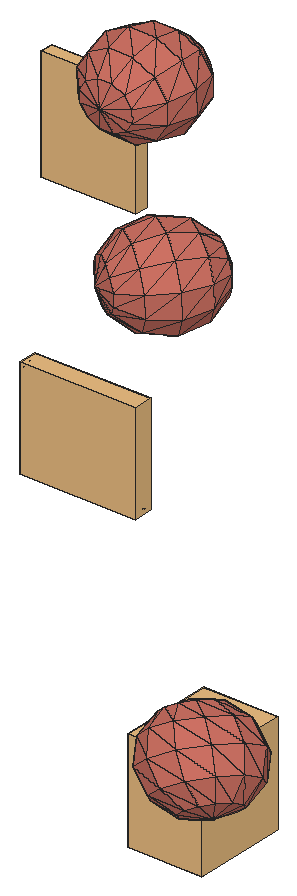
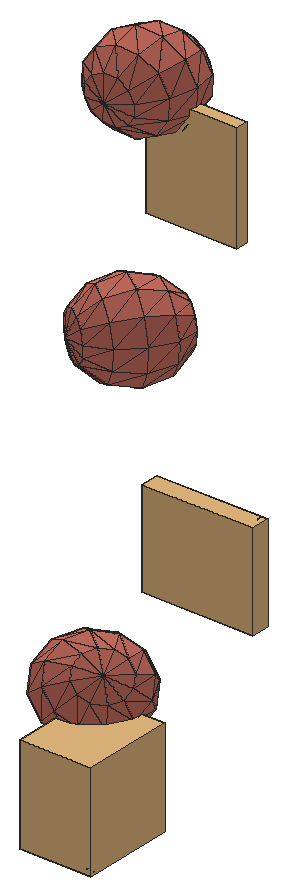
# SketchUp Ruby script. Lengths in inches.
U = 1.inch
M = Sketchup.active_model
def pt(a) = Geom::Point3d.new(a.map { |v| v * U })
def face(e, loops, mat)
  f = e.add_face(loops[0].map { |a| pt(a) })
  loops[1..].each { |l| e.add_face(l.map { |a| pt(a) }).erase! }
  f.material = f.back_material = mat if mat
  f
end
# faces: each face lists its corners as indices into pts; further lists are holes
def faces(e, pts, list, mat = nil) = list.each { |f| face(e, (f[0].is_a?(Array) ? f : [f]).map { |l| l.map { |i| pts[i] } }, mat) }
# xy, xz, yz: faces in a plane at the given z, y or x. An outline is a flat list of corners, or four numbers for a rectangle; further outlines are holes
def ring(l) = l.size == 4 ? [[l[0], l[1]], [l[2], l[1]], [l[2], l[3]], [l[0], l[3]]] : l.each_slice(2).to_a
def flat(e, list, mat, &to3) = list.each { |f| face(e, (f[0].is_a?(Array) ? f : [f]).map { |l| ring(l).map { |u, v| to3.(u, v) } }, mat) }
def xy(e, z, list, mat = nil) = flat(e, list, mat) { |x, y| [x, y, z] }
def xz(e, y, list, mat = nil) = flat(e, list, mat) { |x, z| [x, y, z] }
def yz(e, x, list, mat = nil) = flat(e, list, mat) { |y, z| [x, y, z] }
def lines(e, pts, list) = list.each { |a, b| e.add_line(pt(pts[a]), pt(pts[b])) }
# prism: a flat outline (further loops are holes) pulled along v
def prism(e, loops, v, mat = nil)
  f = face(e, loops, mat); d = Geom::Vector3d.new(v.map { |x| x * U })
  f.pushpull(f.normal.samedirection?(d) ? d.length : -d.length)
end
def box(e, o, s, mat = nil) = prism(e, [[o, [o[0] + s[0], o[1], o[2]], [o[0] + s[0], o[1] + s[1], o[2]], [o[0], o[1] + s[1], o[2]]]], [0, 0, s[2]], mat)
def at(x, y, z, deg = 0) = Geom::Transformation.translation(pt([x, y, z])) * Geom::Transformation.rotation(ORIGIN, Z_AXIS, deg.degrees)
def axes(o, x, y, z) = Geom::Transformation.new([*x, 0, *y, 0, *z, 0, *pt(o).to_a, 1])
def part(name) = M.definitions.add(name)
# library, detail: a bought-in or finely detailed component or shape, given as its bounding box
def library(name, o, s) = part(name).tap { |d| box(d.entities, o, s) }
def detail(e, o, s) = box(e.add_group.entities, o, s)
def put(e, d, t, mat = nil) = e.add_instance(d, t).tap { |i| i.material = mat if mat }
def group(e, t, mat = nil) = e.add_group.tap { |g| g.transformation = t; g.material = mat if mat }.entities
root = M.entities
M.materials.add("green").color = [174, 139, 102]
M.materials.add("vio").color = [206, 114, 100]
c1 = part("3DGeom~245_Defintion")
p = [[84.59,12.79,-493.27],[7.47,-267.01,-389.5],[-107.54,-84.94,-478.67],[229.32,-154.15,-406.37],[223.5,146.29,-413.58],[-82.81,176.3,-448.01],
  [-2.61,253.375,-402],[-216.38,-308.31,-268.27],[-301.4,-120.72,-373.68],[-193.73,119.875,-439.57],[-228.02,292.57,-282.7],[-305.66,99.22,-378.96],
  [389.73,0,-314.35],[271.98,279.79,-260.94],[389.73,0,-314.35],[223.5,146.29,-413.58],[25.38,330.46,-313.87],[271.98,279.79,-260.94],
  [120.48,-377.52,-195.97],[312.61,-279.79,-210.57],[120.48,-377.52,-195.97],[389.73,0,-314.35],[312.61,-279.79,-210.57],[229.32,-154.15,-406.37],
  [7.47,-267.01,-389.5],[-73.38,-413.29,-90.98],[-216.38,-308.31,-268.27],[7.47,-267.01,-389.5],[120.48,-377.52,-195.97],[-305.66,99.22,-378.96],
  [-301.4,-120.72,-373.68],[-445.05,-84.94,-206.44],[-305.66,99.22,-378.96],[-388.6,119.875,-282.4],[-388.6,119.875,-282.4],[-301.4,-120.72,-373.68],
  [-216.38,-308.31,-268.27],[-382.26,-267.01,-75.16],[-301.4,-120.72,-373.68],[389.73,0,-314.35],[451.52,-146.29,-130.88],[312.61,-279.79,-210.57],
  [445.7,154.15,-138.1],[389.73,0,-314.35],[271.98,279.79,-260.94],[389.73,0,-314.35],[-6.34,386.88,-207.25],[271.98,279.79,-260.94],
  [25.38,330.46,-313.87],[25.38,330.46,-313.87],[-228.02,292.57,-282.7],[-420.32,176.3,-175.77],[-228.02,292.57,-282.7],[-392.33,253.375,-87.65],
  [-228.02,292.57,-282.7],[-312.13,330.46,-41.64],[-228.02,292.57,-282.7],[-312.13,330.46,-41.64],[-201.21,386.88,-50.07],[-228.02,292.57,-282.7],
  [-89.28,407.53,-110.6875],[-228.02,292.57,-282.7],[-228.02,292.57,-282.7],[-500,12.79,-21.75],[-216.38,-308.31,-268.27],[-217.03,-377.52,76.26],
  [-216.38,-308.31,-268.27],[-217.03,-377.52,76.26],[-382.26,-267.01,-75.16],[217.03,377.52,-76.26],[271.98,279.79,-260.94],[217.03,377.52,-76.26],
  [271.98,279.79,-260.94],[312.61,-279.79,-210.57],[201.21,-386.88,50.07],[312.61,-279.79,-210.57],[312.13,-330.46,41.64],[312.13,-330.46,41.64],
  [312.61,-279.79,-210.57],[-445.7,-154.15,138.1],[89.28,-407.53,110.6875],[-451.52,146.29,130.88],[500,-12.79,21.75],[382.26,267.01,75.16],
  [217.03,377.52,-76.26],[392.33,-253.375,87.65],[312.13,-330.46,41.64],[73.38,413.29,90.98],[6.34,-386.88,207.25],[-217.03,-377.52,76.26],
  [-312.61,279.79,210.57],[-312.61,279.79,210.57],[-312.13,330.46,-41.64],[382.26,267.01,75.16],[-217.03,-377.52,76.26],[-271.98,-279.79,260.94],
  [-120.48,377.52,195.97],[-312.61,279.79,210.57],[-389.73,0,314.35],[420.32,-176.3,175.78],[445.05,84.94,206.44],[228.02,-292.57,282.7],
  [312.13,-330.46,41.64],[228.02,-292.57,282.7],[216.38,308.31,268.27],[216.38,308.31,268.27],[382.26,267.01,75.16],[-217.03,-377.52,76.26],
  [-25.38,-330.46,313.87],[-217.03,-377.52,76.26],[-25.38,-330.46,313.87],[-271.98,-279.79,260.94],[228.02,-292.57,282.7],[-229.32,154.15,406.37],
  [-229.32,154.15,406.37],[-312.61,279.79,210.57],[-223.5,-146.29,413.58],[-223.5,-146.29,413.58],[388.6,-119.875,282.4],[228.02,-292.57,282.7],
  [-312.61,279.79,210.57],[-7.47,267.01,389.5],[-120.48,377.52,195.97],[-7.47,267.01,389.5],[301.4,120.72,373.68],[216.38,308.31,268.27],
  [-25.38,-330.46,313.87],[-312.61,279.79,210.57],[-229.32,154.15,406.37],[-7.47,267.01,389.5],[-271.98,-279.79,260.94],[-25.38,-330.46,313.87],
  [2.61,-253.375,402],[-271.98,-279.79,260.94],[-223.5,-146.29,413.58],[-7.47,267.01,389.5],[301.4,120.72,373.68],[216.38,308.31,268.27],
  [388.6,-119.875,282.4],[305.66,-99.22,378.96],[228.02,-292.57,282.7],[305.66,-99.22,378.96],[228.02,-292.57,282.7],[82.81,-176.3,448.01],
  [228.02,-292.57,282.7],[193.73,-119.875,439.57],[228.02,-292.57,282.7],[305.66,-99.22,378.96],[228.02,-292.57,282.7],[-389.73,0,314.35],
  [-84.59,-12.79,493.27],[-389.73,0,314.35],[107.54,84.94,478.67],[305.66,-99.22,378.96],[301.4,120.72,373.68],[-7.47,267.01,389.5],
  [301.4,120.72,373.68],[305.66,-99.22,378.96],[-7.47,267.01,389.5]]
faces(c1.entities,p,[[0,1,2],[0,3,1],[4,3,0],[5,0,2],[6,0,5],[6,4,0],[2,7,8],[2,1,7],
  [9,2,8],[5,2,9],[5,9,10],[6,5,10],[9,8,11],[9,11,10],[4,12,3],[13,14,15],
  [16,4,6],[16,17,4],[3,18,1],[3,19,20],[21,22,23],[16,6,10],[24,25,26],[27,28,25],
  [29,30,31],[32,31,33],[11,34,10],[35,36,37],[38,37,31],[39,40,41],[42,40,43],[44,42,45],
  [46,47,48],[46,49,50],[33,51,52],[51,53,54],[53,55,56],[57,58,59],[60,46,61],[58,60,62],
  [33,31,63],[33,63,51],[64,25,65],[66,67,68],[69,42,70],[46,71,72],[73,74,28],[75,76,74],
  [40,77,78],[60,71,46],[31,37,79],[31,79,63],[28,80,25],[28,74,80],[51,63,81],[51,81,53],
  [42,82,40],[83,82,42],[84,83,42],[40,85,86],[82,85,40],[60,87,71],[58,87,60],[25,88,89],
  [25,80,88],[53,81,90],[53,91,92],[87,93,71],[37,94,95],[37,95,79],[57,96,58],[58,96,87],
  [57,97,96],[63,79,98],[63,98,81],[82,99,85],[100,99,82],[83,100,82],[74,76,101],[102,85,103],
  [80,74,101],[104,100,83],[87,105,106],[107,88,108],[109,110,111],[85,99,112],[96,105,87],[88,80,101],
  [81,98,113],[81,114,115],[79,95,116],[79,117,98],[99,118,119],[100,118,99],[120,121,122],[96,123,105],
  [124,118,100],[125,124,100],[126,88,101],[127,128,129],[130,131,132],[133,132,134],[135,136,137],[138,139,140],
  [124,141,118],[132,131,142],[143,132,144],[145,143,146],[147,145,148],[149,134,150],[151,150,128],[152,153,154],
  [155,152,156],[152,145,157],[128,152,158],[134,132,143],[128,150,152],[134,143,150],[150,143,145],[150,145,152]],"vio")
c2 = part("3DGeom~247_Defintion")
p = [[-255.5,94.92,-415.28],[-6.35,103.625,-485.08],[-12.59,-116.1,-481.02],[239.09,-105.72,-421.38],[244.5,84.5625,-424.9],[1.59,295.58,-359.16],
  [-248.62,261.16,-306.23],[-255.5,94.92,-415.28],[-248.62,261.16,-306.23],[-260.91,-95.36,-411.76],[-15.46,-304.71,-348.07],[236.61,-269.07,-306.25],
  [-255.5,94.92,-415.28],[-260.91,-95.36,-411.76],[426.72,-67.02,-248.84],[429.84,42.84,-250.87],[426.72,-67.02,-248.84],[251.38,250.8,-315.85],
  [429.84,42.84,-250.87],[244.5,84.5625,-424.9],[251.38,250.8,-315.85],[239.09,-105.72,-421.38],[425.28,-161.33,-182.37],[236.61,-269.07,-306.25],
  [239.09,-105.72,-421.38],[426.72,-67.02,-248.84],[-436.1875,60.78,-234.21],[-255.5,94.92,-415.28],[-260.91,-95.36,-411.76],[-432.22,156.76,-171.25],
  [-248.62,261.16,-306.23],[-260.91,-95.36,-411.76],[-263.39,-258.71,-296.63],[-439.31,-49.07,-232.18],[-263.39,-258.71,-296.63],[9.11,408.34,-137.01],
  [251.38,250.8,-315.85],[1.59,295.58,-359.16],[-242.11,358.81,-113.84],[1.59,295.58,-359.16],[-248.62,261.16,-306.23],[-242.11,358.81,-113.84],
  [1.59,295.58,-359.16],[-263.39,-258.71,-296.63],[-15.46,-304.71,-348.07],[-14.18,-411.68,-121.86],[-15.46,-304.71,-348.07],[237.72,-361.7,-110.34],
  [-15.46,-304.71,-348.07],[236.61,-269.07,-306.25],[251.38,250.8,-315.85],[433.81,138.82,-187.91],[429.84,42.84,-250.87],[257.89,348.45,-123.46],
  [251.38,250.8,-315.85],[257.89,348.45,-123.46],[251.38,250.8,-315.85],[236.61,-269.07,-306.25],[425.92,-214.8125,-69.26],[237.72,-361.7,-110.34],
  [236.61,-269.07,-306.25],[-428.46,213.14,-60.17],[-242.11,358.81,-113.84],[-263.39,-258.71,-296.63],[-262.28,-351.34,-100.72],[-440.74,-143.38,-165.7],
  [-262.28,-351.34,-100.72],[429.84,42.84,-250.87],[500,-10.36,-9.62],[429.84,42.84,-250.87],[-500,10.36,9.62],[437.57,195.19,-76.83],
  [257.89,348.45,-123.46],[-440.1,-196.87,-52.6],[14.18,411.68,121.86],[-237.72,361.7,110.34],[-242.11,358.81,-113.84],[-237.72,361.7,110.34],
  [262.28,351.34,100.72],[257.89,348.45,-123.46],[262.28,351.34,100.72],[-262.28,-351.34,-100.72],[-9.11,-408.34,137.01],[242.11,-358.81,113.84],
  [-425.92,214.8125,69.26],[-237.72,361.7,110.34],[237.72,-361.7,-110.34],[428.46,-213.14,60.17],[237.72,-361.7,-110.34],[242.11,-358.81,113.84],
  [-262.28,-351.34,-100.72],[-257.89,-348.45,123.46],[-257.89,-348.45,123.46],[440.1,196.87,52.6],[262.28,351.34,100.72],[-437.57,-195.19,76.83],
  [432.22,-156.76,171.25],[436.1875,-60.78,234.21],[439.31,49.07,232.18],[440.74,143.38,165.7],[-433.81,-138.82,187.91],[-429.84,-42.84,250.87],
  [-426.72,67.02,248.84],[-425.28,161.33,182.37],[263.39,258.71,296.63],[263.39,258.71,296.63],[262.28,351.34,100.72],[242.11,-358.81,113.84],
  [-251.38,-250.8,315.85],[15.46,304.71,348.07],[263.39,258.71,296.63],[-236.61,269.07,306.25],[-236.61,269.07,306.25],[-237.72,361.7,110.34],
  [248.62,-261.16,306.23],[242.11,-358.81,113.84],[248.62,-261.16,306.23],[-236.61,269.07,306.25],[-257.89,-348.45,123.46],[-1.59,-295.58,359.16],
  [-257.89,-348.45,123.46],[-1.59,-295.58,359.16],[-251.38,-250.8,315.85],[248.62,-261.16,306.23],[-1.59,-295.58,359.16],[260.91,95.36,411.76],
  [260.91,95.36,411.76],[263.39,258.71,296.63],[248.62,-261.16,306.23],[-244.5,-84.5625,424.9],[-244.5,-84.5625,424.9],[255.5,-94.92,415.28],
  [255.5,-94.92,415.28],[260.91,95.36,411.76],[248.62,-261.16,306.23],[255.5,-94.92,415.28],[-429.84,-42.84,250.87],[-239.09,105.73,421.38],
  [-426.72,67.02,248.84],[-239.09,105.73,421.38],[-429.84,-42.84,250.87],[-244.5,-84.5625,424.9],[-239.09,105.73,421.38],[12.59,116.1,481.02],
  [260.91,95.36,411.76],[263.39,258.71,296.63],[263.39,258.71,296.63],[15.46,304.71,348.07],[-1.59,-295.58,359.16],[248.62,-261.16,306.23],
  [255.5,-94.92,415.28],[-239.09,105.73,421.38],[15.46,304.71,348.07],[-236.61,269.07,306.25],[-251.38,-250.8,315.85],[6.35,-103.625,485.08],
  [-251.38,-250.8,315.85],[-239.09,105.73,421.38],[15.46,304.71,348.07],[-239.09,105.73,421.38]]
faces(c2.entities,p,[[0,1,2],[1,3,2],[1,4,3],[5,4,1],[6,1,7],[8,5,1],[9,2,10],[2,11,10],
  [2,3,11],[12,2,13],[4,14,3],[4,15,16],[17,18,19],[5,20,4],[21,22,23],[24,25,22],
  [26,27,28],[29,27,26],[29,30,27],[31,10,32],[33,28,34],[26,28,33],[35,36,37],[38,39,40],
  [41,35,42],[43,44,45],[46,47,45],[48,49,47],[50,51,52],[53,51,54],[35,55,56],[57,58,59],
  [60,22,58],[61,30,29],[61,62,30],[63,45,64],[65,34,66],[33,34,65],[25,67,68],[69,51,68],
  [22,25,68],[26,33,70],[29,26,70],[33,65,70],[51,71,68],[72,71,51],[58,22,68],[61,29,70],
  [65,66,73],[65,73,70],[74,55,35],[75,35,76],[77,74,35],[78,71,79],[74,80,55],[81,45,82],
  [45,47,83],[45,83,82],[84,62,61],[84,85,62],[86,58,87],[88,87,89],[90,82,91],[73,66,92],
  [71,93,68],[94,93,71],[87,58,68],[84,61,70],[73,92,95],[73,95,70],[96,87,68],[97,96,68],
  [98,97,68],[99,98,68],[93,99,68],[95,100,70],[100,101,70],[101,102,70],[103,84,70],[102,103,70],
  [104,99,93],[105,93,106],[107,87,96],[103,85,84],[95,92,108],[95,108,100],[109,110,80],[109,80,74],
  [103,111,85],[112,74,113],[82,83,114],[115,96,116],[117,109,74],[118,82,119],[120,121,122],[82,123,124],
  [125,98,99],[126,99,127],[128,96,97],[102,111,103],[100,108,129],[100,130,101],[131,97,98],[132,98,133],
  [134,97,135],[136,137,138],[102,139,111],[140,141,142],[143,144,145],[143,146,147],[148,149,150],[151,152,153],
  [154,148,155],[156,155,141],[157,143,158],[148,150,155],[155,150,144],[155,144,143],[141,143,159],[141,155,143]],"vio")
c3 = library("3DGeom~179_Defintion",[-58.28,-500,-420.6],[116.56,1000,841.2])
c4 = part("3DGeom~180_Defintion")
p = [[-21.41,-458.84,-420.6],[-21.53,-500,-365.15],[-53.32,-468.47,-406.125],[10.44,-469.79,-407.35],[-21.53,-500,-365.15],[10.44,-469.79,-407.35],
  [-3.01,-461.98,-417.24],[-53.32,-468.47,-406.125],[-39.83,-461.21,-416.53],[10.38,-490.37,-379.625],[-21.53,-500,-365.15],[10.44,-469.79,-407.35],
  [10.38,-490.37,-379.625],[10.44,-469.79,-407.35],[15.34,-480.18,-393.58],[-53.32,-468.47,-406.125],[-21.53,-500,-365.15],[-53.38,-489.05,-378.4],
  [-53.32,-468.47,-406.125],[-53.38,-489.05,-378.4],[-58.28,-478.66,-392.17],[-21.53,-500,-365.15],[10.38,-490.37,-379.625],[-3.11,-497.625,-369.22],
  [-21.53,-500,-365.15],[-39.93,-496.86,-368.51],[-53.38,-489.05,-378.4],[21.98,487.39,420.6],[20.96,500,348.46],[2.62,499.54,353.65],
  [21.98,487.39,420.6],[39.43,498.77,352.9375],[20.96,500,348.46],[21.98,487.39,420.6],[53.09,496.1875,365.88],[39.43,498.77,352.9375],
  [21.98,487.39,420.6],[2.62,499.54,353.65],[-10.67,497.51,367.11],[21.98,487.39,420.6],[58.28,492.93,383.82],[53.09,496.1875,365.88],
  [21.98,487.39,420.6],[-10.67,497.51,367.11],[-15.34,494.46,385.24],[21.98,487.39,420.6],[53.61,489.88,401.95],[58.28,492.93,383.82],
  [21.98,487.39,420.6],[-15.34,494.46,385.24],[-10.15,491.2,403.18],[21.98,487.39,420.6],[40.32,487.85,415.41],[53.61,489.88,401.95],
  [21.98,487.39,420.6],[-10.15,491.2,403.18],[3.51,488.61,416.12]]
faces(c4.entities,p,[[0,1,2],[3,4,0],[5,0,6],[0,7,8],[9,10,11],[12,13,14],[15,16,17],[18,19,20],
  [21,22,23],[24,25,26],[27,28,29],[30,31,32],[33,34,35],[36,37,38],[39,40,41],[42,43,44],
  [45,46,47],[48,49,50],[51,52,53],[54,55,56]],"green")
c5 = part("3DGeom~217_Defintion")
p = [[-278.9,104.85,-403.93],[-34.22,85.5625,-494.84],[-36.78,-106.97,-488.84],[218.15,-67.8125,-449.7],[219.62,43.35,-453.16],[33.05,253.77,-407.11],
  [-201.22,299.08,-302.625],[-278.9,104.85,-403.93],[-201.22,299.08,-302.625],[-281.85,-117.47,-397],[26.0625,-272.25,-390.72],[254.43,-163.24,-393.05],
  [-278.9,104.85,-403.93],[-281.85,-117.47,-397],[414.62,-10.48,-290.0625],[258.46,140.46,-402.51],[147.02,352.57,-249.16],[-69.62,413.17,-120.23],
  [33.05,253.77,-407.11],[-201.22,299.08,-302.625],[147.02,352.57,-249.16],[33.05,253.77,-407.11],[-448.85,96.04,-204.78],[-278.9,104.85,-403.93],
  [-281.85,-117.47,-397],[-381.57,264.25,-117.05],[-201.22,299.08,-302.625],[258.46,140.46,-402.51],[324.26,197.5,-311.32],[414.62,-10.48,-290.0625],
  [147.02,352.57,-249.16],[324.26,197.5,-311.32],[-451.4,-96.49,-198.78],[-209.29,-308.32,-283.69],[-281.85,-117.47,-397],[-209.29,-308.32,-283.69],
  [318.75,-217.36,-298.39],[318.75,-217.36,-298.39],[254.43,-163.24,-393.05],[414.62,-10.48,-290.0625],[-209.29,-308.32,-283.69],[26.0625,-272.25,-390.72],
  [137.48,-365.99,-226.76],[318.75,-217.36,-298.39],[137.48,-365.99,-226.76],[324.26,197.5,-311.32],[399.39,199.2,-204.01],[414.62,-10.48,-290.0625],
  [277.14,355.5,-63.3],[324.26,197.5,-311.32],[399.39,199.2,-204.01],[324.26,197.5,-311.32],[-267.6,363.06,40.9],[-201.22,299.08,-302.625],
  [-381.57,264.25,-117.05],[-267.6,363.06,40.9],[-201.22,299.08,-302.625],[318.75,-217.36,-298.39],[393.88,-215.66,-191.08],[393.88,-215.66,-191.08],
  [318.75,-217.36,-298.39],[414.62,-10.48,-290.0625],[459.68,-158.62,-99.89],[414.62,-10.48,-290.0625],[498.52,-61.5,-49.24],[414.62,-10.48,-290.0625],
  [500,49.66,-52.7],[414.62,-10.48,-290.0625],[399.39,199.2,-204.01],[463.72,145.08,-109.35],[414.62,-10.48,-290.0625],[414.62,-10.48,-290.0625],
  [-388.56,-261.77,-100.65],[-209.29,-308.32,-283.69],[-80.64,-416.55,-94.37],[-209.29,-308.32,-283.69],[-388.56,-261.77,-100.65],[80.64,416.55,94.37],
  [267.6,-363.06,-40.9],[393.88,-215.66,-191.08],[-498.52,61.5,49.24],[-459.68,158.62,99.89],[388.56,261.77,100.65],[399.39,199.2,-204.01],
  [388.56,261.77,100.65],[399.39,199.2,-204.01],[277.14,355.5,-63.3],[-500,-49.66,52.7],[267.6,-363.06,-40.9],[-137.48,365.99,226.76],
  [-267.6,363.06,40.9],[-393.88,215.66,191.08],[-267.6,363.06,40.9],[451.4,96.49,198.78],[388.56,261.77,100.65],[-388.56,-261.77,-100.65],
  [-277.14,-355.5,63.3],[-463.72,-145.08,109.35],[-277.14,-355.5,63.3],[267.6,-363.06,-40.9],[381.57,-264.25,117.05],[69.62,-413.17,120.23],
  [209.29,308.32,283.69],[388.56,261.77,100.65],[448.85,-96.04,204.78],[381.57,-264.25,117.05],[-318.75,217.36,298.39],[-267.6,363.06,40.9],
  [-393.88,215.66,191.08],[-318.75,217.36,298.39],[-267.6,363.06,40.9],[-414.62,10.48,290.0625],[-147.02,-352.57,249.16],[-277.14,-355.5,63.3],
  [-399.39,-199.2,204.01],[-399.39,-199.2,204.01],[-147.02,-352.57,249.16],[-26.0625,272.25,390.72],[-26.0625,272.25,390.72],[281.85,117.47,397],
  [388.56,261.77,100.65],[281.85,117.47,397],[388.56,261.77,100.65],[209.29,308.32,283.69],[381.57,-264.25,117.05],[201.22,-299.08,302.625],
  [201.22,-299.08,302.625],[-147.02,-352.57,249.16],[201.22,-299.08,302.625],[-318.75,217.36,298.39],[278.9,-104.85,403.93],[278.9,-104.85,403.93],
  [281.85,117.47,397],[-399.39,-199.2,204.01],[-147.02,-352.57,249.16],[-324.26,-197.5,311.32],[-324.26,-197.5,311.32],[201.22,-299.08,302.625],
  [278.9,-104.85,403.93],[-254.43,163.24,393.05],[-137.48,365.99,226.76],[-318.75,217.36,298.39],[-254.43,163.24,393.05],[-26.0625,272.25,390.72],
  [-137.48,365.99,226.76],[-324.26,-197.5,311.32],[-147.02,-352.57,249.16],[-33.05,-253.77,407.11],[-147.02,-352.57,249.16],[201.22,-299.08,302.625],
  [-33.05,-253.77,407.11],[36.78,106.98,488.84],[209.29,308.32,283.69],[281.85,117.47,397],[209.29,308.32,283.69],[-258.46,-140.46,402.51],
  [-258.46,-140.46,402.51],[-219.62,-43.35,453.16],[-414.62,10.48,290.0625],[-218.15,67.8125,449.7],[-414.62,10.48,290.0625],[-254.43,163.24,393.05],
  [-254.43,163.24,393.05],[-414.62,10.48,290.0625],[201.22,-299.08,302.625],[278.9,-104.85,403.93],[-324.26,-197.5,311.32],[-254.43,163.24,393.05],
  [34.22,-85.5625,494.84]]
faces(c5.entities,p,[[0,1,2],[1,3,2],[1,4,3],[5,4,1],[6,1,7],[8,5,1],[9,2,10],[2,11,10],
  [2,3,11],[12,2,13],[3,4,14],[4,15,14],[5,15,4],[11,3,14],[16,15,5],[17,18,19],
  [17,20,21],[22,23,24],[25,23,22],[25,26,23],[27,28,29],[30,31,15],[32,24,33],[34,10,35],
  [22,24,32],[10,11,36],[37,38,39],[40,41,42],[10,43,44],[45,46,47],[48,49,20],[48,50,51],
  [52,53,54],[55,17,56],[42,57,58],[59,60,61],[62,59,63],[64,62,65],[66,64,67],[68,69,70],
  [69,66,71],[72,73,74],[75,42,74],[32,33,76],[77,20,17],[77,48,20],[74,42,78],[42,79,78],
  [80,22,32],[81,22,80],[81,25,22],[82,69,83],[84,85,86],[87,32,76],[80,32,87],[88,59,62],
  [89,17,90],[89,77,17],[91,25,81],[91,92,25],[93,66,69],[93,69,94],[95,74,96],[97,76,98],
  [87,76,97],[99,62,100],[100,62,64],[96,74,101],[74,78,101],[102,103,48],[102,48,77],[104,64,66],
  [104,66,93],[100,64,104],[101,78,105],[106,107,108],[109,89,110],[80,87,111],[81,80,111],[87,97,111],
  [96,101,112],[97,113,114],[115,96,116],[117,77,89],[118,102,77],[91,81,111],[119,93,120],[121,122,123],
  [97,114,111],[101,124,125],[126,100,104],[127,101,128],[129,91,111],[130,104,93],[131,93,132],[133,134,135],
  [114,136,111],[137,104,138],[139,140,141],[142,143,144],[145,146,147],[148,149,150],[151,152,143],[151,153,154],
  [136,155,111],[156,157,158],[157,159,160],[161,129,111],[159,162,163],[147,164,165],[166,147,156],[159,143,167],
  [159,151,143],[168,165,153],[168,153,151],[156,147,168],[156,168,157],[147,165,168],[157,151,159],[157,168,151]],"vio")
c6 = library("3DGeom~175_Defintion",[-468.83,-500,-365.63],[937.66,1000,731.26])
c7 = part("3DGeom~176_Defintion")
p = [[-400.83,-477.04,-357.55],[-432.9,-455.37,-364.27],[-414.5,-464.73,-365.63],[-400.83,-477.04,-357.55],[-463.57,-474.42,-303.18],[-432.9,-455.37,-364.27],
  [-432.9,-455.37,-364.27],[-463.57,-474.42,-303.18],[-464.27,-454.05,-337.08],[-432.9,-455.37,-364.27],[-464.27,-454.05,-337.08],[-451.12,-451.46,-353.82],
  [-400.14,-497.41,-323.65],[-463.57,-474.42,-303.18],[-400.83,-477.04,-357.55],[-400.14,-497.41,-323.65],[-400.83,-477.04,-357.55],[-395.58,-489,-342.18],
  [-463.57,-474.42,-303.18],[-468.83,-462.46,-318.55],[-464.27,-454.05,-337.08],[-431.5,-496.09,-296.46],[-400.14,-497.41,-323.65],[-413.29,-500,-306.91],
  [-431.5,-496.09,-296.46],[-463.57,-474.42,-303.18],[-400.14,-497.41,-323.65],[-463.57,-474.42,-303.18],[-431.5,-496.09,-296.46],[-449.91,-486.73,-295.09],
  [426,485.85,358.46],[461.26,458.37,290.55],[449.4375,472.35,283.375],[426,485.85,358.46],[449.4375,472.35,283.375],[436.0625,486.26,287.22],
  [426,485.85,358.46],[436.0625,486.26,287.22],[424.71,496.38,301.05],[426,485.85,358.46],[468.35,448.07,306.83],[461.26,458.37,290.55],
  [426,485.85,358.46],[424.71,496.38,301.05],[418.43,500,321.17],[426,485.85,358.46],[468.83,444.22,327.84],[468.35,448.07,306.83],
  [426,485.85,358.46],[418.43,500,321.17],[418.9,496.14,342.18],[426,485.85,358.46],[462.55,447.84,347.96],[468.83,444.22,327.84],
  [426,485.85,358.46],[451.2,457.96,361.79],[462.55,447.84,347.96],[426,485.85,358.46],[437.82,471.87,365.63],[451.2,457.96,361.79]]
faces(c7.entities,p,[[0,1,2],[3,4,5],[6,7,8],[9,10,11],[12,13,14],[15,16,17],[18,19,20],[21,22,23],
  [24,25,26],[27,28,29],[30,31,32],[33,34,35],[36,37,38],[39,40,41],[42,43,44],[45,46,47],
  [48,49,50],[51,52,53],[54,55,56],[57,58,59]],"green")
c8 = library("3DGeom~167_Defintion",[-82.54,-434.125,-500],[165.09,868.26,1000])
c9 = part("3DGeom~168_Defintion")
p = [[25.15,421.84,-478.96],[-0.29,388.84,-500],[-17.78,385.7,-494.64],[25.15,421.84,-478.96],[15.1875,397.625,-498.65],[-0.29,388.84,-500],
  [25.15,421.84,-478.96],[24.5,409.7,-490.95],[25.15,421.84,-478.96],[-17.78,385.7,-494.64],[-32.61,389.04,-484],[25.15,421.84,-478.96],
  [-32.61,389.04,-484],[-40.79,397.98,-470.93],[25.15,421.84,-478.96],[-40.79,397.98,-470.93],[-40.14,410.12,-458.94],[25.15,421.84,-478.96],
  [-40.14,410.12,-458.94],[-30.83,422.2,-451.24],[25.15,421.84,-478.96],[-30.83,422.2,-451.24],[-15.35,430.99,-449.89],[25.15,421.84,-478.96],
  [-15.35,430.99,-449.89],[2.14,434.13,-455.26],[25.15,421.84,-478.96],[2.14,434.13,-455.26],[16.97,430.78,-465.89],[-23.73,-430.73,456.61],
  [-58.59,-431.87,447.46],[-40.15,-434.125,448.67],[-58.59,-431.87,447.46],[-12.82,-411.91,482.88],[-82.54,-414.19,464.58],[-58.59,-431.87,447.46],
  [-82.54,-414.19,464.58],[-74.11,-424.57,453.28],[-23.73,-430.73,456.61],[-12.82,-411.91,482.88],[-58.59,-431.87,447.46],[-12.82,-411.91,482.88],
  [-23.73,-430.73,456.61],[-13.73,-422.6,469.125],[-82.54,-414.19,464.58],[-12.82,-411.91,482.88],[-71.64,-395.37,490.85],[-82.54,-414.19,464.58],
  [-81.64,-403.5,478.33],[-12.82,-411.91,482.88],[-36.78,-394.23,500],[-12.82,-411.91,482.88],[-21.26,-401.53,494.18],[-55.22,-391.98,498.78]]
faces(c9.entities,p,[[0,1,2],[3,4,5],[6,7,4],[8,9,10],[11,12,13],[14,15,16],[17,18,19],[20,21,22],
  [23,24,25],[26,27,28],[29,30,31],[32,33,34],[35,36,37],[38,39,40],[41,42,43],[44,45,46],
  [47,46,48],[46,49,50],[51,52,50],[46,50,53]],"green")
g1 = group(root,at(15.3125,38.42,26.21))
put(g1,c1,axes([-0.58,-0.43,11.25],[0,0.00039,0],[0,0,-0.00039],[-0.00039,0,0]),"vio")
g2 = group(root,at(15.3125,38.42,26.21))
put(g2,c2,axes([-0.78,-0.43,13.33],[0,0.00039,0],[0,0,-0.00039],[-0.00039,0,0]),"vio")
g3 = group(root,at(15.3125,38.42,26.21))
put(g3,c3,axes([-0.97,-0.42,13.11],[0,0.0004,0],[0,0,-0.0004],[-0.0004,0,0]),"green")
put(g3,c4,axes([-0.97,-0.42,13.11],[0,0.0004,0],[0,0,-0.0004],[-0.0004,0,0]),"green")
g4 = group(root,at(15.3125,38.42,26.21))
put(g4,c5,axes([-0.86,-0.25,12.61],[0,0.00039,0],[0,0,-0.00039],[-0.00039,0,0]),"vio")
g5 = group(root,at(15.3125,38.42,26.21))
put(g5,c6,axes([-0.72,-0.25,11.05],[0,0.00036,0],[0,0,-0.00036],[-0.00036,0,0]),"green")
put(g5,c7,axes([-0.72,-0.25,11.05],[0,0.00036,0],[0,0,-0.00036],[-0.00036,0,0]),"green")
g6 = group(root,at(15.3125,38.42,26.21))
put(g6,c8,axes([-1.16,-0.22,11.98],[0,0.00041,0],[0,0,-0.00041],[-0.00041,0,0]),"green")
put(g6,c9,axes([-1.16,-0.22,11.98],[0,0.00041,0],[0,0,-0.00041],[-0.00041,0,0]),"green")
